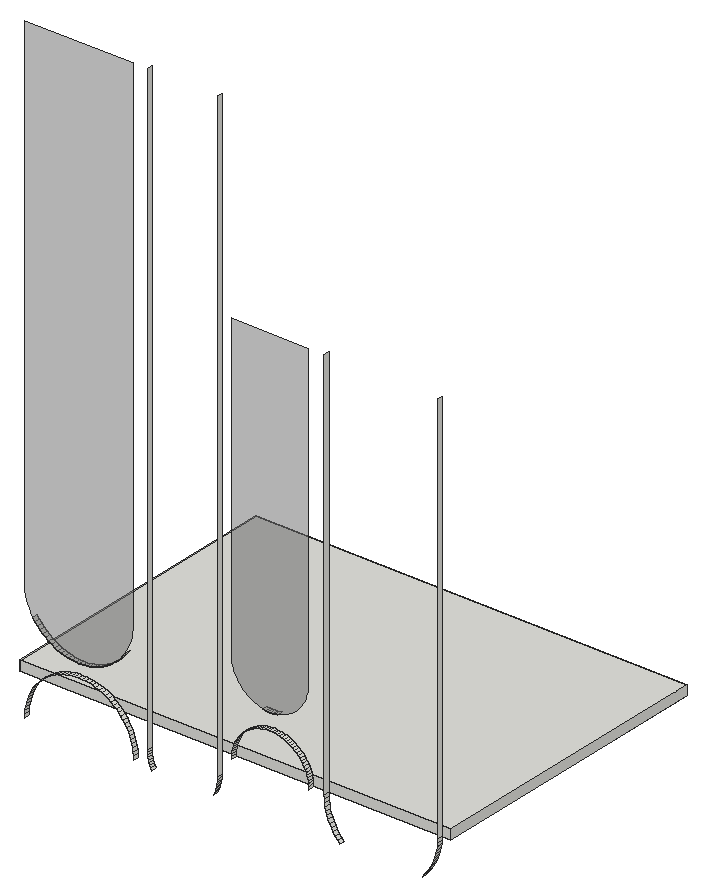
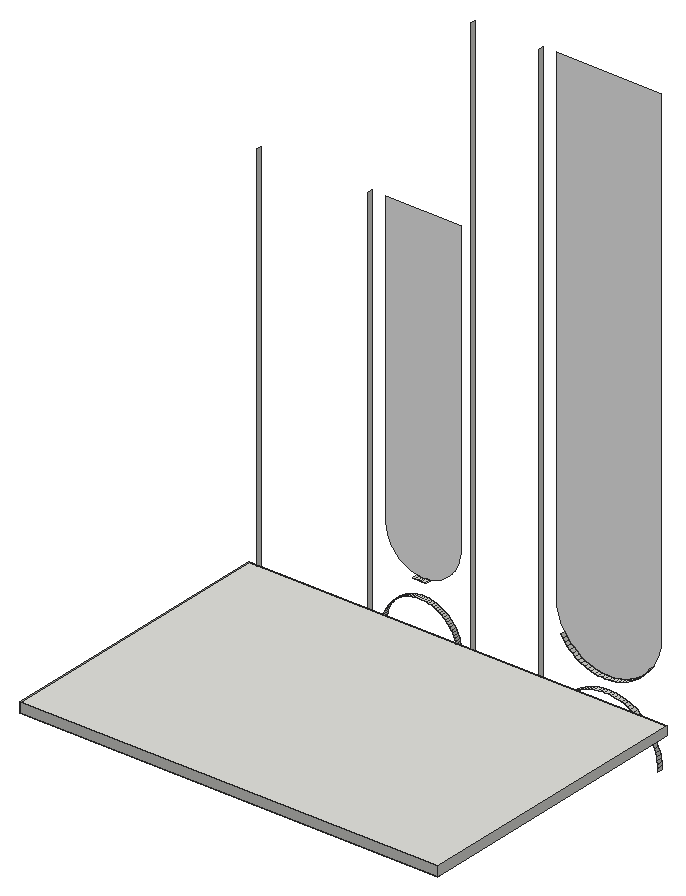
# SketchUp Ruby script. Lengths in inches.
U = 1.inch
M = Sketchup.active_model
def pt(a) = Geom::Point3d.new(a.map { |v| v * U })
def face(e, loops, mat)
  f = e.add_face(loops[0].map { |a| pt(a) })
  loops[1..].each { |l| e.add_face(l.map { |a| pt(a) }).erase! }
  f.material = f.back_material = mat if mat
  f
end
# faces: each face lists its corners as indices into pts; further lists are holes
def faces(e, pts, list, mat = nil) = list.each { |f| face(e, (f[0].is_a?(Array) ? f : [f]).map { |l| l.map { |i| pts[i] } }, mat) }
# xy, xz, yz: faces in a plane at the given z, y or x. An outline is a flat list of corners, or four numbers for a rectangle; further outlines are holes
def ring(l) = l.size == 4 ? [[l[0], l[1]], [l[2], l[1]], [l[2], l[3]], [l[0], l[3]]] : l.each_slice(2).to_a
def flat(e, list, mat, &to3) = list.each { |f| face(e, (f[0].is_a?(Array) ? f : [f]).map { |l| ring(l).map { |u, v| to3.(u, v) } }, mat) }
def xy(e, z, list, mat = nil) = flat(e, list, mat) { |x, y| [x, y, z] }
def xz(e, y, list, mat = nil) = flat(e, list, mat) { |x, z| [x, y, z] }
def yz(e, x, list, mat = nil) = flat(e, list, mat) { |y, z| [x, y, z] }
def lines(e, pts, list) = list.each { |a, b| e.add_line(pt(pts[a]), pt(pts[b])) }
# prism: a flat outline (further loops are holes) pulled along v
def prism(e, loops, v, mat = nil)
  f = face(e, loops, mat); d = Geom::Vector3d.new(v.map { |x| x * U })
  f.pushpull(f.normal.samedirection?(d) ? d.length : -d.length)
end
def box(e, o, s, mat = nil) = prism(e, [[o, [o[0] + s[0], o[1], o[2]], [o[0] + s[0], o[1] + s[1], o[2]], [o[0], o[1] + s[1], o[2]]]], [0, 0, s[2]], mat)
def at(x, y, z, deg = 0) = Geom::Transformation.translation(pt([x, y, z])) * Geom::Transformation.rotation(ORIGIN, Z_AXIS, deg.degrees)
def axes(o, x, y, z) = Geom::Transformation.new([*x, 0, *y, 0, *z, 0, *pt(o).to_a, 1])
def part(name) = M.definitions.add(name)
# library, detail: a bought-in or finely detailed component or shape, given as its bounding box
def library(name, o, s) = part(name).tap { |d| box(d.entities, o, s) }
def detail(e, o, s) = box(e.add_group.entities, o, s)
def put(e, d, t, mat = nil) = e.add_instance(d, t).tap { |i| i.material = mat if mat }
def group(e, t, mat = nil) = e.add_group.tap { |g| g.transformation = t; g.material = mat if mat }.entities
root = M.entities
M.materials.add("[Translucent Glass Gray]").color = [128, 128, 128]
M.materials["[Translucent Glass Gray]"].alpha = 0.5
c1 = part("Group\#2")
box(c1.entities,[0,0,0],[753.47,516,17])
xz(root,487.08,[[1590.02,418.51,1596.4,418.72,1602.76,419.36,1609.06,420.42,1615.27,421.9,1621.375,423.78,1627.34,426.07,1633.14,428.76,1638.74,431.82,1644.13,435.25,1649.28,439.03,1654.17,443.14,1658.77,447.57,1663.0625,452.3,1667.03,457.31,1670.66,462.5625,1673.93,468.05,1676.83,473.74,1679.34,479.62,1681.46,485.64,1683.17,491.8,1684.46,498.05,1685.34,504.38,1685.42,505.5,1685.42,1394,1494.625,1394,1494.625,505.5,1494.7,504.38,1495.58,498.05,1496.875,491.8,1498.58,485.64,1500.7,479.62,1503.21,473.74,1506.11,468.05,1509.38,462.5625,1513.01,457.31,1516.98,452.3,1521.27,447.57,1525.875,443.14,1530.76,439.03,1535.91,435.25,1541.3,431.82,1546.9,428.76,1552.7,426.07,1558.66,423.78,1564.77,421.9,1570.98,420.42,1577.28,419.36,1583.64,418.72],[1924.64,459.07,1928.91,459.21,1933.16,459.61,1937.37,460.27,1941.54,461.21,1945.64,462.4,1949.65,463.84,1953.57,465.54,1957.37,467.47,1961.04,469.65,1964.57,472.04,1967.94,474.66,1971.14,477.48,1974.16,480.5,1976.98,483.7,1979.6,487.07,1982,490.6,1984.17,494.28,1986.11,498.08,1987.8,501.99,1989.25,506.01,1990.4375,510.11,1991.37,514.27,1992.04,518.49,1992.4375,522.73,1992.57,527,1992.57,1054,1856.72,1054,1856.72,527,1856.85,522.73,1857.25,518.49,1857.92,514.27,1858.85,510.11,1860.04,506.01,1861.49,501.99,1863.18,498.08,1865.12,494.28,1867.29,490.6,1869.6875,487.07,1872.3,483.7,1875.125,480.5,1878.14,477.48,1881.35,474.66,1884.72,472.04,1888.25,469.65,1891.92,467.47,1895.72,465.54,1899.64,463.84,1903.65,462.4,1907.75,461.21,1911.92,460.27,1916.13,459.61,1920.38,459.21]],"[Translucent Glass Gray]")
yz(root,1709.42,[[487.08,325.5,496.08,1394]])
yz(root,1832.72,[[487.08,325.5,496.08,1394]])
yz(root,2019.16,[[487.08,364.18,496.08,1054]])
yz(root,2218.1,[[487.08,364.18,496.08,1054]])
p = [[1715.28,487.08,299.25],[1717.04,487.08,295.8],[1717.04,496.08,295.8],[1715.28,496.08,299.25],[1825.09,487.08,295.8],[1826.85,487.08,299.25],
  [1826.85,496.08,299.25],[1825.09,496.08,295.8],[2041.98,487.08,300.77],[2046.12,487.08,296.08],[2046.12,496.08,296.08],[2041.98,496.08,300.77],
  [2191.14,487.08,296.08],[2195.27,487.08,300.77],[2195.27,496.08,300.77],[2191.14,496.08,296.08],[1713.75,487.08,302.8],[1713.75,496.08,302.8],
  [1828.39,487.08,302.8],[1828.39,496.08,302.8],[1494.8125,487.08,306.78],[1494.625,487.08,300.79],[1494.625,496.08,300.79],[1494.8125,496.08,306.78],
  [1685.42,487.08,300.79],[1685.23,487.08,306.78],[1685.23,496.08,306.78],[1685.42,496.08,300.79],[2038.15,487.08,305.71],[2038.15,496.08,305.71],
  [2199.1,487.08,305.71],[2199.1,496.08,305.71],[1712.43,487.08,306.45],[1712.43,496.08,306.45],[1829.7,487.08,306.45],[1829.7,496.08,306.45],
  [2034.64,487.08,310.88],[2034.64,496.08,310.88],[2202.61,487.08,310.88],[2202.61,496.08,310.88],[1711.35,487.08,310.17],[1711.35,496.08,310.17],
  [1830.78,487.08,310.17],[1830.78,496.08,310.17],[1495.375,487.08,312.74],[1495.375,496.08,312.74],[1684.66,487.08,312.74],[1684.66,496.08,312.74],
  [1710.51,487.08,313.95],[1710.51,496.08,313.95],[1831.625,487.08,313.95],[1831.625,496.08,313.95],[2031.46,487.08,316.26],[2031.46,496.08,316.26],
  [2205.79,487.08,316.26],[2205.79,496.08,316.26],[1496.3125,487.08,318.66],[1496.3125,496.08,318.66],[1683.73,487.08,318.66],[1683.73,496.08,318.66],
  [1709.9,487.08,317.77],[1709.9,496.08,317.77],[1832.23,487.08,317.77],[1832.23,496.08,317.77],[2028.62,487.08,321.82],[2028.62,496.08,321.82],
  [2208.63,487.08,321.82],[2208.63,496.08,321.82],[1709.54,487.08,321.63],[1709.54,496.08,321.63],[1832.59,487.08,321.63],[1832.59,496.08,321.63],
  [1497.62,487.08,324.51],[1497.62,496.08,324.51],[1682.42,487.08,324.51],[1682.42,496.08,324.51],[1709.42,487.08,325.5],[1709.42,496.08,325.5],
  [1832.72,487.08,325.5],[1832.72,496.08,325.5],[2026.14,487.08,327.56],[2026.14,496.08,327.56],[2211.11,487.08,327.56],[2211.11,496.08,327.56],
  [1499.29,487.08,330.27],[1499.29,496.08,330.27],[1680.75,487.08,330.27],[1680.75,496.08,330.27],[2024.02,487.08,333.4375],[2024.02,496.08,333.4375],
  [2213.23,487.08,333.4375],[2213.23,496.08,333.4375],[1501.32,487.08,335.9],[1501.32,496.08,335.9],[1678.72,487.08,335.9],[1678.72,496.08,335.9],
  [2022.28,487.08,339.4375],[2022.28,496.08,339.4375],[2214.97,487.08,339.4375],[2214.97,496.08,339.4375],[1503.7,487.08,341.4],[1503.7,496.08,341.4],
  [1676.34,487.08,341.4],[1676.34,496.08,341.4],[2020.92,487.08,345.54],[2020.92,496.08,345.54],[2216.34,487.08,345.54],[2216.34,496.08,345.54],
  [1506.42,487.08,346.74],[1506.42,496.08,346.74],[1673.62,487.08,346.74],[1673.62,496.08,346.74],[2019.94,487.08,351.71],[2019.94,496.08,351.71],
  [2217.3125,487.08,351.71],[2217.3125,496.08,351.71],[1509.47,487.08,351.9],[1509.47,496.08,351.9],[1670.57,487.08,351.9],[1670.57,496.08,351.9],
  [2019.35,487.08,357.93],[2019.35,496.08,357.93],[2217.9,487.08,357.93],[2217.9,496.08,357.93],[1512.84,487.08,356.86],[1512.84,496.08,356.86],
  [1667.2,487.08,356.86],[1667.2,496.08,356.86],[1516.52,487.08,361.59],[1516.52,496.08,361.59],[1663.52,487.08,361.59],[1663.52,496.08,361.59],
  [2019.16,487.08,364.18],[2019.16,496.08,364.18],[2218.1,487.08,364.18],[2218.1,496.08,364.18],[1520.48,487.08,366.09],[1520.48,496.08,366.09],
  [1659.5625,487.08,366.09],[1659.5625,496.08,366.09],[1856.85,487.08,366.99],[1856.72,487.08,362.73],[1856.72,496.08,362.73],[1856.85,496.08,366.99],
  [1992.57,487.08,362.73],[1992.4375,487.08,366.99],[1992.4375,496.08,366.99],[1992.57,496.08,362.73],[1524.72,487.08,370.33],[1524.72,496.08,370.33],
  [1655.32,487.08,370.33],[1655.32,496.08,370.33],[1857.25,487.08,371.24],[1857.25,496.08,371.24],[1992.04,487.08,371.24],[1992.04,496.08,371.24],
  [1529.21,487.08,374.29],[1529.21,496.08,374.29],[1650.83,487.08,374.29],[1650.83,496.08,374.29],[1857.92,487.08,375.46],[1857.92,496.08,375.46],
  [1991.37,487.08,375.46],[1991.37,496.08,375.46],[1533.95,487.08,377.96],[1533.95,496.08,377.96],[1646.09,487.08,377.96],[1646.09,496.08,377.96],
  [1858.85,487.08,379.62],[1858.85,496.08,379.62],[1990.4375,487.08,379.62],[1990.4375,496.08,379.62],[1538.9,487.08,381.33],[1538.9,496.08,381.33],
  [1641.14,487.08,381.33],[1641.14,496.08,381.33],[1860.04,487.08,383.72],[1860.04,496.08,383.72],[1989.25,487.08,383.72],[1989.25,496.08,383.72],
  [1544.0625,487.08,384.38],[1544.0625,496.08,384.38],[1635.98,487.08,384.38],[1635.98,496.08,384.38],[1861.49,487.08,387.74],[1861.49,496.08,387.74],
  [1987.8,487.08,387.74],[1987.8,496.08,387.74],[1549.4,487.08,387.1],[1549.4,496.08,387.1],[1630.64,487.08,387.1],[1630.64,496.08,387.1],
  [1554.9,487.08,389.48],[1554.9,496.08,389.48],[1625.14,487.08,389.48],[1625.14,496.08,389.48],[1863.18,487.08,391.65],[1863.18,496.08,391.65],
  [1986.11,487.08,391.65],[1986.11,496.08,391.65],[1560.54,487.08,391.51],[1560.54,496.08,391.51],[1619.5,487.08,391.51],[1619.5,496.08,391.51],
  [1566.3,487.08,393.1875],[1566.3,496.08,393.1875],[1613.74,487.08,393.1875],[1613.74,496.08,393.1875],[1865.12,487.08,395.45],[1865.12,496.08,395.45],
  [1984.17,487.08,395.45],[1984.17,496.08,395.45],[1572.14,487.08,394.49],[1572.14,496.08,394.49],[1607.9,487.08,394.49],[1607.9,496.08,394.49],
  [1578.0625,487.08,395.43],[1578.0625,496.08,395.43],[1601.98,487.08,395.43],[1601.98,496.08,395.43],[1584.03,487.08,395.99],[1584.03,496.08,395.99],
  [1596.01,487.08,395.99],[1596.01,496.08,395.99],[1867.29,487.08,399.13],[1867.29,496.08,399.13],[1982,487.08,399.13],[1982,496.08,399.13],
  [1590.02,487.08,396.18],[1590.02,496.08,396.18],[1869.6875,487.08,402.66],[1869.6875,496.08,402.66],[1979.6,487.08,402.66],[1979.6,496.08,402.66],
  [1872.3,487.08,406.03],[1872.3,496.08,406.03],[1976.98,487.08,406.03],[1976.98,496.08,406.03],[1875.125,487.08,409.23],[1875.125,496.08,409.23],
  [1974.16,487.08,409.23],[1974.16,496.08,409.23],[1878.14,487.08,412.25],[1878.14,496.08,412.25],[1971.14,487.08,412.25],[1971.14,496.08,412.25],
  [1881.35,487.08,415.07],[1881.35,496.08,415.07],[1967.94,487.08,415.07],[1967.94,496.08,415.07],[1884.72,487.08,417.68],[1884.72,496.08,417.68],
  [1964.57,487.08,417.68],[1964.57,496.08,417.68],[1888.25,487.08,420.08],[1888.25,496.08,420.08],[1961.04,487.08,420.08],[1961.04,496.08,420.08],
  [1583.64,487.08,418.72],[1590.02,487.08,418.51],[1590.02,496.08,418.51],[1583.64,496.08,418.72],[1596.4,487.08,418.72],[1596.4,496.08,418.72],
  [1577.28,487.08,419.36],[1577.28,496.08,419.36],[1602.76,487.08,419.36],[1602.76,496.08,419.36],[1570.98,487.08,420.42],[1570.98,496.08,420.42],
  [1609.06,487.08,420.42],[1609.06,496.08,420.42],[1891.92,487.08,422.26],[1891.92,496.08,422.26],[1957.37,487.08,422.26],[1957.37,496.08,422.26],
  [1564.77,487.08,421.9],[1564.77,496.08,421.9],[1615.27,487.08,421.9],[1615.27,496.08,421.9],[1558.66,487.08,423.78],[1558.66,496.08,423.78],
  [1621.375,487.08,423.78],[1621.375,496.08,423.78],[1895.72,487.08,424.19],[1895.72,496.08,424.19],[1957.125,487.08,422.38],[1957.125,496.08,422.38],
  [1953.57,496.08,424.19],[1953.57,487.08,424.19],[1552.7,487.08,426.07],[1552.7,496.08,426.07],[1627.34,487.08,426.07],[1627.34,496.08,426.07],
  [1899.64,487.08,425.89],[1899.64,496.08,425.89],[1949.65,487.08,425.89],[1949.65,496.08,425.89],[1903.65,487.08,427.33],[1903.65,496.08,427.33],
  [1945.64,487.08,427.33],[1945.64,496.08,427.33],[1546.9,487.08,428.76],[1546.9,496.08,428.76],[1633.14,487.08,428.76],[1633.14,496.08,428.76],
  [1907.75,487.08,428.52],[1907.75,496.08,428.52],[1941.54,487.08,428.52],[1941.54,496.08,428.52],[1911.92,487.08,429.45],[1911.92,496.08,429.45],
  [1937.37,487.08,429.45],[1937.37,496.08,429.45],[1541.3,487.08,431.82],[1541.3,496.08,431.82],[1638.74,487.08,431.82],[1638.74,496.08,431.82],
  [1916.13,487.08,430.12],[1916.13,496.08,430.12],[1933.16,487.08,430.12],[1933.16,496.08,430.12],[1920.38,487.08,430.52],[1920.38,496.08,430.52],
  [1928.91,487.08,430.52],[1928.91,496.08,430.52],[1924.64,487.08,430.66],[1924.64,496.08,430.66],[1535.91,487.08,435.25],[1535.91,496.08,435.25],
  [1644.13,487.08,435.25],[1644.13,496.08,435.25],[1530.76,487.08,439.03],[1530.76,496.08,439.03],[1649.28,487.08,439.03],[1649.28,496.08,439.03],
  [1525.875,487.08,443.14],[1525.875,496.08,443.14],[1654.17,487.08,443.14],[1654.17,496.08,443.14],[1521.27,487.08,447.57],[1521.27,496.08,447.57],
  [1658.77,487.08,447.57],[1658.77,496.08,447.57],[1516.98,487.08,452.3],[1516.98,496.08,452.3],[1663.0625,487.08,452.3],[1663.0625,496.08,452.3],
  [1513.01,487.08,457.31],[1513.01,496.08,457.31],[1667.03,487.08,457.31],[1667.03,496.08,457.31],[1509.38,487.08,462.5625],[1509.38,496.08,462.5625],
  [1670.66,487.08,462.5625],[1670.66,496.08,462.5625],[1920.38,487.08,459.21],[1924.64,487.08,459.07],[1924.64,496.08,459.07],[1920.38,496.08,459.21],
  [1928.91,487.08,459.21],[1928.91,496.08,459.21],[1916.13,487.08,459.61],[1916.13,496.08,459.61],[1933.16,487.08,459.61],[1933.16,496.08,459.61],
  [1911.92,487.08,460.27],[1911.92,496.08,460.27],[1937.37,487.08,460.27],[1937.37,496.08,460.27]]
faces(root,p,[[0,1,2,3],[4,5,6,7],[8,9,10,11],[12,13,14,15],[16,0,3,17],[5,18,19,6],[20,21,22,23],[24,25,26,27],
  [28,8,11,29],[13,30,31,14],[32,16,17,33],[18,34,35,19],[36,28,29,37],[30,38,39,31],[40,32,33,41],[34,42,43,35],
  [44,20,23,45],[25,46,47,26],[48,40,41,49],[42,50,51,43],[52,36,37,53],[38,54,55,39],[56,44,45,57],[46,58,59,47],
  [60,48,49,61],[50,62,63,51],[64,52,53,65],[54,66,67,55],[68,60,61,69],[62,70,71,63],[72,56,57,73],[58,74,75,59],
  [76,68,69,77],[70,78,79,71],[80,64,65,81],[66,82,83,67],[84,72,73,85],[74,86,87,75],[88,80,81,89],[82,90,91,83],
  [92,84,85,93],[86,94,95,87],[96,88,89,97],[90,98,99,91],[100,92,93,101],[94,102,103,95],[104,96,97,105],[98,106,107,99],
  [108,100,101,109],[102,110,111,103],[112,104,105,113],[106,114,115,107],[116,108,109,117],[110,118,119,111],[120,112,113,121],[114,122,123,115],
  [124,116,117,125],[118,126,127,119],[128,124,125,129],[126,130,131,127],[132,120,121,133],[122,134,135,123],[136,128,129,137],[130,138,139,131],
  [140,141,142,143],[144,145,146,147],[148,136,137,149],[138,150,151,139],[152,140,143,153],[145,154,155,146],[156,148,149,157],[150,158,159,151],
  [160,152,153,161],[154,162,163,155],[164,156,157,165],[158,166,167,159],[168,160,161,169],[162,170,171,163],[172,164,165,173],[166,174,175,167],
  [176,168,169,177],[170,178,179,171],[180,172,173,181],[174,182,183,175],[184,176,177,185],[178,186,187,179],[188,180,181,189],[182,190,191,183],
  [192,188,189,193],[190,194,195,191],[196,184,185,197],[186,198,199,187],[200,192,193,201],[194,202,203,195],[204,200,201,205],[202,206,207,203],
  [208,196,197,209],[198,210,211,199],[212,204,205,213],[206,214,215,207],[216,212,213,217],[214,218,219,215],[220,216,217,221],[218,222,223,219],
  [224,208,209,225],[210,226,227,211],[228,220,221,229],[222,228,229,223],[230,224,225,231],[226,232,233,227],[234,230,231,235],[232,236,237,233],
  [238,234,235,239],[236,240,241,237],[242,238,239,243],[240,244,245,241],[246,242,243,247],[244,248,249,245],[250,246,247,251],[248,252,253,249],
  [254,250,251,255],[252,256,257,253],[258,259,260,261],[259,262,263,260],[264,258,261,265],[262,266,267,263],[268,264,265,269],[266,270,271,267],
  [272,254,255,273],[256,274,275,257],[276,268,269,277],[270,278,279,271],[280,276,277,281],[278,282,283,279],[284,272,273,285],[274,286,287,275],
  [288,287,286,289],[290,280,281,291],[282,292,293,283],[294,284,285,295],[289,296,297,288],[298,294,295,299],[296,300,301,297],[302,290,291,303],
  [292,304,305,293],[306,298,299,307],[300,308,309,301],[310,306,307,311],[308,312,313,309],[314,302,303,315],[304,316,317,305],[318,310,311,319],
  [312,320,321,313],[322,318,319,323],[320,324,325,321],[326,322,323,327],[324,326,327,325],[328,314,315,329],[316,330,331,317],[332,328,329,333],
  [330,334,335,331],[336,332,333,337],[334,338,339,335],[340,336,337,341],[338,342,343,339],[344,340,341,345],[342,346,347,343],[348,344,345,349],
  [346,350,351,347],[352,348,349,353],[350,354,355,351],[356,357,358,359],[357,360,361,358],[362,356,359,363],[360,364,365,361],[366,362,363,367],
  [364,368,369,365]])
put(root,c1,at(1479.625,496.08,364.18))
